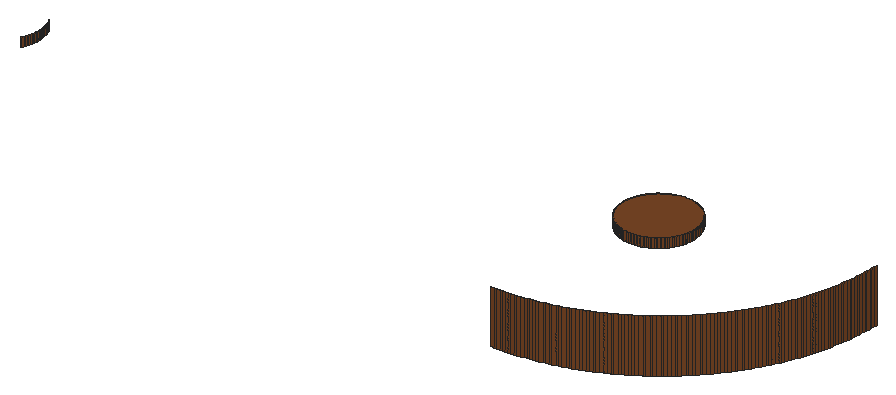
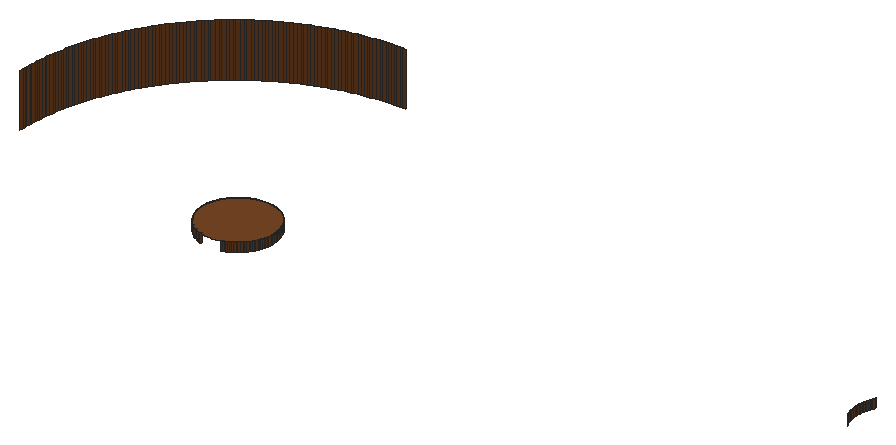
# SketchUp Ruby script. Lengths in inches.
U = 1.inch
M = Sketchup.active_model
def pt(a) = Geom::Point3d.new(a.map { |v| v * U })
def face(e, loops, mat)
  f = e.add_face(loops[0].map { |a| pt(a) })
  loops[1..].each { |l| e.add_face(l.map { |a| pt(a) }).erase! }
  f.material = f.back_material = mat if mat
  f
end
# faces: each face lists its corners as indices into pts; further lists are holes
def faces(e, pts, list, mat = nil) = list.each { |f| face(e, (f[0].is_a?(Array) ? f : [f]).map { |l| l.map { |i| pts[i] } }, mat) }
# xy, xz, yz: faces in a plane at the given z, y or x. An outline is a flat list of corners, or four numbers for a rectangle; further outlines are holes
def ring(l) = l.size == 4 ? [[l[0], l[1]], [l[2], l[1]], [l[2], l[3]], [l[0], l[3]]] : l.each_slice(2).to_a
def flat(e, list, mat, &to3) = list.each { |f| face(e, (f[0].is_a?(Array) ? f : [f]).map { |l| ring(l).map { |u, v| to3.(u, v) } }, mat) }
def xy(e, z, list, mat = nil) = flat(e, list, mat) { |x, y| [x, y, z] }
def xz(e, y, list, mat = nil) = flat(e, list, mat) { |x, z| [x, y, z] }
def yz(e, x, list, mat = nil) = flat(e, list, mat) { |y, z| [x, y, z] }
def lines(e, pts, list) = list.each { |a, b| e.add_line(pt(pts[a]), pt(pts[b])) }
# prism: a flat outline (further loops are holes) pulled along v
def prism(e, loops, v, mat = nil)
  f = face(e, loops, mat); d = Geom::Vector3d.new(v.map { |x| x * U })
  f.pushpull(f.normal.samedirection?(d) ? d.length : -d.length)
end
def box(e, o, s, mat = nil) = prism(e, [[o, [o[0] + s[0], o[1], o[2]], [o[0] + s[0], o[1] + s[1], o[2]], [o[0], o[1] + s[1], o[2]]]], [0, 0, s[2]], mat)
def at(x, y, z, deg = 0) = Geom::Transformation.translation(pt([x, y, z])) * Geom::Transformation.rotation(ORIGIN, Z_AXIS, deg.degrees)
def axes(o, x, y, z) = Geom::Transformation.new([*x, 0, *y, 0, *z, 0, *pt(o).to_a, 1])
def part(name) = M.definitions.add(name)
# library, detail: a bought-in or finely detailed component or shape, given as its bounding box
def library(name, o, s) = part(name).tap { |d| box(d.entities, o, s) }
def detail(e, o, s) = box(e.add_group.entities, o, s)
def put(e, d, t, mat = nil) = e.add_instance(d, t).tap { |i| i.material = mat if mat }
def group(e, t, mat = nil) = e.add_group.tap { |g| g.transformation = t; g.material = mat if mat }.entities
root = M.entities
M.materials.add("[Wood Veneer 01]3").color = [120, 70, 37]
xy(root,118.5,[[142.9,38,142.74,38.02,142.65,38.03,142.41,38.09,142.17,38.18,142.1,38.21,142.02,38.25,141.95,38.3,141.88,38.34,141.8125,38.39,141.75,38.44,141.68,38.5,141.62,38.55,141.5625,38.61,141.5,38.67,141.45,38.74,141.4,38.8,141.3,38.94,141.26,39.01,141.22,39.09,141.18,39.16,141.09,39.4,141.03,39.64,141.01,39.8,141,39.89,141,40.14,141.01,40.22,141.02,40.31,141.1,40.63,141.16,40.79,141.2,40.86,141.23,40.9375,141.27,41.01,141.47,41.29,141.52,41.35,141.64,41.47,141.7,41.52,141.77,41.58,141.84,41.625,141.9,41.67,141.98,41.72,142.05,41.76,142.125,41.8,142.2,41.83,142.44,41.92,142.6,41.96,142.68,41.97,142.76,41.99,142.85,41.99,142.93,42,143.1,42,143.26,41.98,143.35,41.97,143.59,41.91,143.83,41.82,143.9,41.79,143.98,41.75,144.05,41.7,144.12,41.66,144.1875,41.61,144.25,41.56,144.32,41.5,144.38,41.45,144.4375,41.39,144.5,41.33,144.55,41.26,144.6,41.2,144.7,41.06,144.74,40.99,144.78,40.91,144.82,40.84,144.91,40.6,144.97,40.36,144.99,40.2,145,40.11,145,39.86,144.99,39.78,144.98,39.69,144.9,39.37,144.84,39.21,144.8,39.14,144.77,39.0625,144.73,38.99,144.53,38.71,144.48,38.65,144.36,38.53,144.3,38.48,144.23,38.42,144.16,38.375,144.1,38.33,144.02,38.28,143.95,38.24,143.875,38.2,143.8,38.17,143.56,38.08,143.4,38.04,143.32,38.03,143.24,38.01,143.15,38.01,143.07,38]],"[Wood Veneer 01]3")
xz(root,27,[[144,118,144.16,121],[144.16,118,144.3125,121]],"[Wood Veneer 01]3")
xz(root,38,[[142.9,118,142.99,118.5],[142.99,118,143.07,118.5]],"[Wood Veneer 01]3")
xz(root,38.01,[[143.15,118,143.24,118.5]],"[Wood Veneer 01]3")
yz(root,111.5,[[35.86,118,35.94,118.5],[35.94,118,36.03,118.5],[36.03,118,36.11,118.5]],"[Wood Veneer 01]3")
yz(root,141,[[39.89,118,39.97,118.5],[39.97,118,40.06,118.5],[40.06,118,40.14,118.5]],"[Wood Veneer 01]3")
yz(root,145,[[39.86,118,39.94,118.5],[39.94,118,40.03,118.5],[40.03,118,40.11,118.5]],"[Wood Veneer 01]3")
yz(root,156,[[38.6875,118,38.84,121],[38.84,118,39,121]],"[Wood Veneer 01]3")
p = [[144.47,27.01,121],[144.3125,27,121],[144.3125,27,118],[144.47,27.01,118],[144.63,27.02,121],[144.63,27.02,118],
  [144.78,27.03,121],[144.78,27.03,118],[144.94,27.04,121],[144.94,27.04,118],[145.1,27.05,121],[145.1,27.05,118],
  [145.25,27.07,121],[145.25,27.07,118],[145.41,27.08,121],[145.41,27.08,118],[145.57,27.1,121],[145.57,27.1,118],
  [145.72,27.125,121],[145.72,27.125,118],[145.88,27.15,121],[145.88,27.15,118],[146.03,27.17,121],[146.03,27.17,118],
  [146.1875,27.2,121],[146.1875,27.2,118],[146.34,27.23,121],[146.34,27.23,118],[146.49,27.26,121],[146.49,27.26,118],
  [146.65,27.3,121],[146.65,27.3,118],[146.8,27.33,121],[146.8,27.33,118],[146.95,27.37,121],[146.95,27.37,118],
  [147.11,27.41,121],[147.11,27.41,118],[147.26,27.45,121],[147.26,27.45,118],[147.41,27.49,121],[147.41,27.49,118],
  [147.56,27.54,121],[147.56,27.54,118],[147.71,27.59,121],[147.71,27.59,118],[147.86,27.64,121],[147.86,27.64,118],
  [148.01,27.6875,121],[148.01,27.6875,118],[148.15,27.74,121],[148.15,27.74,118],[148.3,27.8,121],[148.3,27.8,118],
  [148.45,27.85,121],[148.45,27.85,118],[148.59,27.91,121],[148.59,27.91,118],[148.74,27.97,121],[148.74,27.97,118],
  [148.88,28.04,121],[148.88,28.04,118],[149.02,28.1,121],[149.02,28.1,118],[149.17,28.17,121],[149.17,28.17,118],
  [149.31,28.24,121],[149.31,28.24,118],[149.45,28.31,121],[149.45,28.31,118],[149.59,28.38,121],[149.59,28.38,118],
  [149.73,28.45,121],[149.73,28.45,118],[149.86,28.53,121],[149.86,28.53,118],[150,28.61,121],[150,28.61,118],
  [150.14,28.6875,121],[150.14,28.6875,118],[150.27,28.77,121],[150.27,28.77,118],[150.4,28.85,121],[150.4,28.85,118],
  [150.54,28.9375,121],[150.54,28.9375,118],[150.67,29.02,121],[150.67,29.02,118],[150.8,29.11,121],[150.8,29.11,118],
  [150.93,29.2,121],[150.93,29.2,118],[151.05,29.29,121],[151.05,29.29,118],[151.18,29.38,121],[151.18,29.38,118],
  [151.31,29.48,121],[151.31,29.48,118],[151.43,29.58,121],[151.43,29.58,118],[151.55,29.67,121],[151.55,29.67,118],
  [151.67,29.77,121],[151.67,29.77,118],[151.79,29.875,121],[151.79,29.875,118],[151.91,29.98,121],[151.91,29.98,118],
  [152.03,30.08,121],[152.03,30.08,118],[152.15,30.1875,121],[152.15,30.1875,118],[152.26,30.3,121],[152.26,30.3,118],
  [152.375,30.4,121],[152.375,30.4,118],[152.49,30.51,121],[152.49,30.51,118],[152.6,30.625,121],[152.6,30.625,118],
  [152.7,30.74,121],[152.7,30.74,118],[152.8125,30.85,121],[152.8125,30.85,118],[152.92,30.97,121],[152.92,30.97,118],
  [153.02,31.09,121],[153.02,31.09,118],[153.125,31.21,121],[153.125,31.21,118],[153.23,31.33,121],[153.23,31.33,118],
  [153.33,31.45,121],[153.33,31.45,118],[153.42,31.57,121],[153.42,31.57,118],[153.52,31.69,121],[153.52,31.69,118],
  [153.62,31.82,121],[153.62,31.82,118],[153.71,31.95,121],[153.71,31.95,118],[153.8,32.07,121],[153.8,32.07,118],
  [153.89,32.2,121],[153.89,32.2,118],[153.98,32.33,121],[153.98,32.33,118],[154.0625,32.46,121],[154.0625,32.46,118],
  [154.15,32.6,121],[154.15,32.6,118],[154.23,32.73,121],[154.23,32.73,118],[154.3125,32.86,121],[154.3125,32.86,118],
  [154.39,33,121],[154.39,33,118],[154.47,33.14,121],[154.47,33.14,118],[154.55,33.27,121],[154.55,33.27,118],
  [154.62,33.41,121],[154.62,33.41,118],[154.69,33.55,121],[154.69,33.55,118],[154.76,33.69,121],[154.76,33.69,118],
  [154.83,33.83,121],[154.83,33.83,118],[154.9,33.98,121],[154.9,33.98,118],[154.96,34.12,121],[154.96,34.12,118],
  [155.03,34.26,121],[155.03,34.26,118],[155.09,34.41,121],[155.09,34.41,118],[155.15,34.55,121],[155.15,34.55,118],
  [155.2,34.7,121],[155.2,34.7,118],[155.26,34.85,121],[155.26,34.85,118],[155.3125,34.99,121],[155.3125,34.99,118],
  [111.27,35.0625,118],[111.23,34.99,118],[111.23,34.99,118.5],[111.27,35.0625,118.5],[155.36,35.14,121],[155.36,35.14,118],
  [111.3,35.14,118],[111.3,35.14,118.5],[111.34,35.21,118],[111.34,35.21,118.5],[155.41,35.29,121],[155.41,35.29,118],
  [111.37,35.29,118],[111.37,35.29,118.5],[111.4,35.37,118],[111.4,35.37,118.5],[155.46,35.44,121],[155.46,35.44,118],
  [111.42,35.45,118],[111.42,35.45,118.5],[111.44,35.53,118],[111.44,35.53,118.5],[155.51,35.59,121],[155.51,35.59,118],
  [111.46,35.61,118],[111.46,35.61,118.5],[111.48,35.69,118],[111.48,35.69,118.5],[155.55,35.74,121],[155.55,35.74,118],
  [111.49,35.78,118],[111.49,35.78,118.5],[155.59,35.89,121],[155.59,35.89,118],[111.5,35.86,118],[111.5,35.86,118.5],
  [155.63,36.05,121],[155.63,36.05,118],[155.67,36.2,121],[155.67,36.2,118],[111.49,36.2,118],[111.5,36.11,118],
  [111.5,36.11,118.5],[111.49,36.2,118.5],[111.48,36.28,118],[111.48,36.28,118.5],[155.7,36.35,121],[155.7,36.35,118],
  [111.47,36.36,118],[111.47,36.36,118.5],[111.43,36.52,118],[111.45,36.44,118],[111.45,36.44,118.5],[111.43,36.52,118.5],
  [155.74,36.51,121],[155.74,36.51,118],[111.41,36.6,118],[111.41,36.6,118.5],[155.77,36.66,121],[155.77,36.66,118],
  [111.38,36.68,118],[111.38,36.68,118.5],[111.35,36.76,118],[111.35,36.76,118.5],[155.8,36.8125,121],[155.8,36.8125,118],
  [111.32,36.84,118],[111.32,36.84,118.5],[111.28,36.91,118],[111.28,36.91,118.5],[155.83,36.97,121],[155.83,36.97,118],
  [111.24,36.99,118],[111.24,36.99,118.5],[155.85,37.12,121],[155.85,37.12,118],[155.875,37.28,121],[155.875,37.28,118],
  [155.9,37.43,121],[155.9,37.43,118],[155.92,37.59,121],[155.92,37.59,118],[155.93,37.75,121],[155.93,37.75,118],
  [155.95,37.9,121],[155.95,37.9,118],[155.96,38.06,121],[155.96,38.06,118],[142.57,38.05,118],[142.49,38.07,118],
  [142.49,38.07,118.5],[142.57,38.05,118.5],[142.65,38.03,118],[142.65,38.03,118.5],[142.82,38.01,118],[142.74,38.02,118],
  [142.74,38.02,118.5],[142.82,38.01,118.5],[142.9,38,118],[142.9,38,118.5],[143.15,38.01,118],[143.07,38,118],
  [143.07,38,118.5],[143.15,38.01,118.5],[143.32,38.03,118],[143.24,38.01,118],[143.24,38.01,118.5],[143.32,38.03,118.5],
  [143.4,38.04,118],[143.4,38.04,118.5],[143.48,38.06,118],[143.48,38.06,118.5],[142.25,38.15,118],[142.17,38.18,118],
  [142.17,38.18,118.5],[142.25,38.15,118.5],[142.41,38.09,118],[142.33,38.12,118],[142.33,38.12,118.5],[142.41,38.09,118.5],
  [143.56,38.08,118],[143.56,38.08,118.5],[143.64,38.11,118],[143.64,38.11,118.5],[143.72,38.14,118],[143.72,38.14,118.5],
  [143.8,38.17,118],[143.8,38.17,118.5],[155.97,38.22,121],[155.97,38.22,118],[142.1,38.21,118],[142.02,38.25,118],
  [142.02,38.25,118.5],[142.1,38.21,118.5],[143.875,38.2,118],[143.875,38.2,118.5],[143.95,38.24,118],[143.95,38.24,118.5],
  [144.02,38.28,118],[144.02,38.28,118.5],[155.98,38.37,121],[155.98,38.37,118],[141.88,38.34,118],[141.8125,38.39,118],
  [141.8125,38.39,118.5],[141.88,38.34,118.5],[141.95,38.3,118],[141.95,38.3,118.5],[144.1,38.33,118],[144.1,38.33,118.5],
  [144.16,38.375,118],[144.16,38.375,118.5],[141.75,38.44,118],[141.75,38.44,118.5],[141.68,38.5,118],[141.68,38.5,118.5],
  [144.23,38.42,118],[144.23,38.42,118.5],[144.3,38.48,118],[144.3,38.48,118.5],[155.99,38.53,121],[155.99,38.53,118],
  [141.62,38.55,118],[141.62,38.55,118.5],[144.36,38.53,118],[144.36,38.53,118.5],[144.42,38.59,118],[144.42,38.59,118.5],
  [156,38.6875,121],[156,38.6875,118],[141.5625,38.61,118],[141.5,38.67,118],[141.5,38.67,118.5],[141.5625,38.61,118.5],
  [144.48,38.65,118],[144.48,38.65,118.5],[141.45,38.74,118],[141.4,38.8,118],[141.4,38.8,118.5],[141.45,38.74,118.5],
  [144.53,38.71,118],[144.53,38.71,118.5],[144.58,38.78,118],[144.58,38.78,118.5],[141.35,38.87,118],[141.35,38.87,118.5],
  [144.63,38.85,118],[144.63,38.85,118.5],[144.68,38.92,118],[144.68,38.92,118.5],[141.3,38.94,118],[141.3,38.94,118.5],
  [141.26,39.01,118],[141.26,39.01,118.5],[144.73,38.99,118],[144.73,38.99,118.5],[141.22,39.09,118],[141.22,39.09,118.5],
  [144.77,39.0625,118],[144.77,39.0625,118.5],[141.18,39.16,118],[141.18,39.16,118.5],[144.8,39.14,118],[144.8,39.14,118.5],
  [144.84,39.21,118],[144.84,39.21,118.5],[141.15,39.24,118],[141.12,39.32,118],[141.12,39.32,118.5],[141.15,39.24,118.5],
  [144.87,39.29,118],[144.87,39.29,118.5],[141.09,39.4,118],[141.09,39.4,118.5],[144.9,39.37,118],[144.9,39.37,118.5],
  [141.07,39.48,118],[141.07,39.48,118.5],[144.92,39.45,118],[144.92,39.45,118.5],[144.94,39.53,118],[144.94,39.53,118.5],
  [141.05,39.56,118],[141.05,39.56,118.5],[144.96,39.61,118],[144.96,39.61,118.5],[141.03,39.64,118],[141.03,39.64,118.5],
  [141.02,39.72,118],[141.02,39.72,118.5],[144.98,39.69,118],[144.98,39.69,118.5],[141.01,39.8,118],[141.01,39.8,118.5],
  [144.99,39.78,118],[144.99,39.78,118.5],[141,39.89,118],[141,39.89,118.5],[145,39.86,118],[145,39.86,118.5],
  [141,40.14,118],[141.01,40.22,118],[141.01,40.22,118.5],[141,40.14,118.5],[144.99,40.2,118],[145,40.11,118],
  [145,40.11,118.5],[144.99,40.2,118.5],[141.02,40.31,118],[141.02,40.31,118.5],[144.98,40.28,118],[144.98,40.28,118.5],
  [141.04,40.39,118],[141.04,40.39,118.5],[144.97,40.36,118],[144.97,40.36,118.5],[141.06,40.47,118],[141.06,40.47,118.5],
  [144.93,40.52,118],[144.95,40.44,118],[144.95,40.44,118.5],[144.93,40.52,118.5],[141.08,40.55,118],[141.08,40.55,118.5],
  [144.91,40.6,118],[144.91,40.6,118.5],[141.1,40.63,118],[141.1,40.63,118.5],[141.13,40.71,118],[141.13,40.71,118.5],
  [144.88,40.68,118],[144.88,40.68,118.5],[141.16,40.79,118],[141.16,40.79,118.5],[144.85,40.76,118],[144.85,40.76,118.5],
  [141.2,40.86,118],[141.2,40.86,118.5],[144.82,40.84,118],[144.82,40.84,118.5],[144.78,40.91,118],[144.78,40.91,118.5],
  [141.23,40.9375,118],[141.23,40.9375,118.5],[141.27,41.01,118],[141.27,41.01,118.5],[144.74,40.99,118],[144.74,40.99,118.5],
  [141.32,41.08,118],[141.32,41.08,118.5],[144.7,41.06,118],[144.7,41.06,118.5],[141.37,41.15,118],[141.37,41.15,118.5],
  [144.6,41.2,118],[144.65,41.13,118],[144.65,41.13,118.5],[144.6,41.2,118.5],[141.42,41.22,118],[141.42,41.22,118.5],
  [141.47,41.29,118],[141.47,41.29,118.5],[144.55,41.26,118],[144.55,41.26,118.5],[141.52,41.35,118],[141.52,41.35,118.5],
  [141.58,41.41,118],[141.58,41.41,118.5],[144.4375,41.39,118],[144.5,41.33,118],[144.5,41.33,118.5],[144.4375,41.39,118.5],
  [141.64,41.47,118],[141.64,41.47,118.5],[144.32,41.5,118],[144.38,41.45,118],[144.38,41.45,118.5],[144.32,41.5,118.5],
  [141.7,41.52,118],[141.7,41.52,118.5],[141.77,41.58,118],[141.77,41.58,118.5],[144.25,41.56,118],[144.25,41.56,118.5],
  [141.84,41.625,118],[141.84,41.625,118.5],[141.9,41.67,118],[141.9,41.67,118.5],[144.12,41.66,118],[144.1875,41.61,118],
  [144.1875,41.61,118.5],[144.12,41.66,118.5],[141.98,41.72,118],[141.98,41.72,118.5],[142.05,41.76,118],[142.05,41.76,118.5],
  [143.9,41.79,118],[143.98,41.75,118],[143.98,41.75,118.5],[143.9,41.79,118.5],[144.05,41.7,118],[144.05,41.7,118.5],
  [142.125,41.8,118],[142.125,41.8,118.5],[142.2,41.83,118],[142.2,41.83,118.5],[142.28,41.86,118],[142.28,41.86,118.5],
  [143.75,41.85,118],[143.83,41.82,118],[143.83,41.82,118.5],[143.75,41.85,118.5],[142.36,41.89,118],[142.36,41.89,118.5],
  [142.44,41.92,118],[142.44,41.92,118.5],[143.51,41.93,118],[143.59,41.91,118],[143.59,41.91,118.5],[143.51,41.93,118.5],
  [143.67,41.88,118],[143.67,41.88,118.5]]
faces(root,p,[[0,1,2,3],[4,0,3,5],[6,4,5,7],[8,6,7,9],[10,8,9,11],[12,10,11,13],[14,12,13,15],[16,14,15,17],
  [18,16,17,19],[20,18,19,21],[22,20,21,23],[24,22,23,25],[26,24,25,27],[28,26,27,29],[30,28,29,31],[32,30,31,33],
  [34,32,33,35],[36,34,35,37],[38,36,37,39],[40,38,39,41],[42,40,41,43],[44,42,43,45],[46,44,45,47],[48,46,47,49],
  [50,48,49,51],[52,50,51,53],[54,52,53,55],[56,54,55,57],[58,56,57,59],[60,58,59,61],[62,60,61,63],[64,62,63,65],
  [66,64,65,67],[68,66,67,69],[70,68,69,71],[72,70,71,73],[74,72,73,75],[76,74,75,77],[78,76,77,79],[80,78,79,81],
  [82,80,81,83],[84,82,83,85],[86,84,85,87],[88,86,87,89],[90,88,89,91],[92,90,91,93],[94,92,93,95],[96,94,95,97],
  [98,96,97,99],[100,98,99,101],[102,100,101,103],[104,102,103,105],[106,104,105,107],[108,106,107,109],[110,108,109,111],[112,110,111,113],
  [114,112,113,115],[116,114,115,117],[118,116,117,119],[120,118,119,121],[122,120,121,123],[124,122,123,125],[126,124,125,127],[128,126,127,129],
  [130,128,129,131],[132,130,131,133],[134,132,133,135],[136,134,135,137],[138,136,137,139],[140,138,139,141],[142,140,141,143],[144,142,143,145],
  [146,144,145,147],[148,146,147,149],[150,148,149,151],[152,150,151,153],[154,152,153,155],[156,154,155,157],[158,156,157,159],[160,158,159,161],
  [162,160,161,163],[164,162,163,165],[166,164,165,167],[168,166,167,169],[170,168,169,171],[172,170,171,173],[174,172,173,175],[176,174,175,177],
  [178,176,177,179],[180,178,179,181],[182,180,181,183],[184,182,183,185],[186,187,188,189],[190,184,185,191],[192,186,189,193],[194,192,193,195],
  [196,190,191,197],[198,194,195,199],[200,198,199,201],[202,196,197,203],[204,200,201,205],[206,204,205,207],[208,202,203,209],[210,206,207,211],
  [212,210,211,213],[214,208,209,215],[216,212,213,217],[218,214,215,219],[220,216,217,221],[222,218,219,223],[224,222,223,225],[226,227,228,229],
  [230,226,229,231],[232,224,225,233],[234,230,231,235],[236,237,238,239],[237,234,235,238],[240,232,233,241],[242,236,239,243],[244,240,241,245],
  [246,242,243,247],[248,246,247,249],[250,244,245,251],[252,248,249,253],[254,252,253,255],[256,250,251,257],[258,254,255,259],[260,256,257,261],
  [262,260,261,263],[264,262,263,265],[266,264,265,267],[268,266,267,269],[270,268,269,271],[272,270,271,273],[274,275,276,277],[278,274,277,279],
  [280,281,282,283],[281,278,279,282],[284,280,283,285],[286,287,288,289],[290,291,292,293],[294,290,293,295],[296,294,295,297],[298,299,300,301],
  [302,303,304,305],[303,298,301,304],[275,302,305,276],[306,296,297,307],[308,306,307,309],[310,308,309,311],[312,310,311,313],[314,272,273,315],
  [316,317,318,319],[299,316,319,300],[320,312,313,321],[322,320,321,323],[324,322,323,325],[326,314,315,327],[328,329,330,331],[332,328,331,333],
  [317,332,333,318],[334,324,325,335],[336,334,335,337],[329,338,339,330],[338,340,341,339],[342,336,337,343],[344,342,343,345],[346,326,327,347],
  [340,348,349,341],[350,344,345,351],[352,350,351,353],[354,346,347,355],[356,357,358,359],[348,356,359,349],[360,352,353,361],[362,363,364,365],
  [357,362,365,358],[366,360,361,367],[368,366,367,369],[363,370,371,364],[372,368,369,373],[374,372,373,375],[370,376,377,371],[376,378,379,377],
  [380,374,375,381],[378,382,383,379],[384,380,381,385],[382,386,387,383],[388,384,385,389],[390,388,389,391],[392,393,394,395],[386,392,395,387],
  [396,390,391,397],[393,398,399,394],[400,396,397,401],[398,402,403,399],[404,400,401,405],[406,404,405,407],[402,408,409,403],[410,406,407,411],
  [408,412,413,409],[412,414,415,413],[416,410,411,417],[414,418,419,415],[420,416,417,421],[418,422,423,419],[424,420,421,425],[426,427,428,429],
  [430,431,432,433],[427,434,435,428],[436,430,433,437],[434,438,439,435],[440,436,437,441],[438,442,443,439],[444,445,446,447],[445,440,441,446],
  [442,448,449,443],[450,444,447,451],[448,452,453,449],[452,454,455,453],[456,450,451,457],[454,458,459,455],[460,456,457,461],[458,462,463,459],
  [464,460,461,465],[466,464,465,467],[462,468,469,463],[468,470,471,469],[472,466,467,473],[470,474,475,471],[476,472,473,477],[474,478,479,475],
  [480,481,482,483],[481,476,477,482],[478,484,485,479],[484,486,487,485],[488,480,483,489],[486,490,491,487],[490,492,493,491],[494,495,496,497],
  [495,488,489,496],[492,498,499,493],[500,501,502,503],[501,494,497,502],[498,504,505,499],[504,506,507,505],[508,500,503,509],[506,510,511,507],
  [510,512,513,511],[514,515,516,517],[515,508,509,516],[512,518,519,513],[518,520,521,519],[522,523,524,525],[526,514,517,527],[523,526,527,524],
  [520,528,529,521],[528,530,531,529],[530,532,533,531],[534,535,536,537],[535,522,525,536],[532,538,539,533],[538,540,541,539],[542,543,544,545],
  [543,546,547,544],[546,534,537,547]],"[Wood Veneer 01]3")
